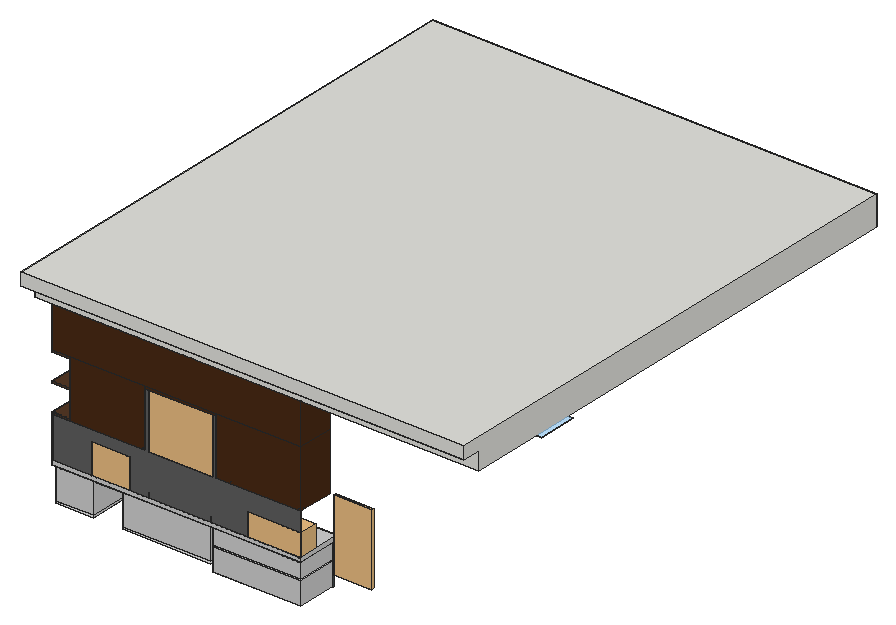
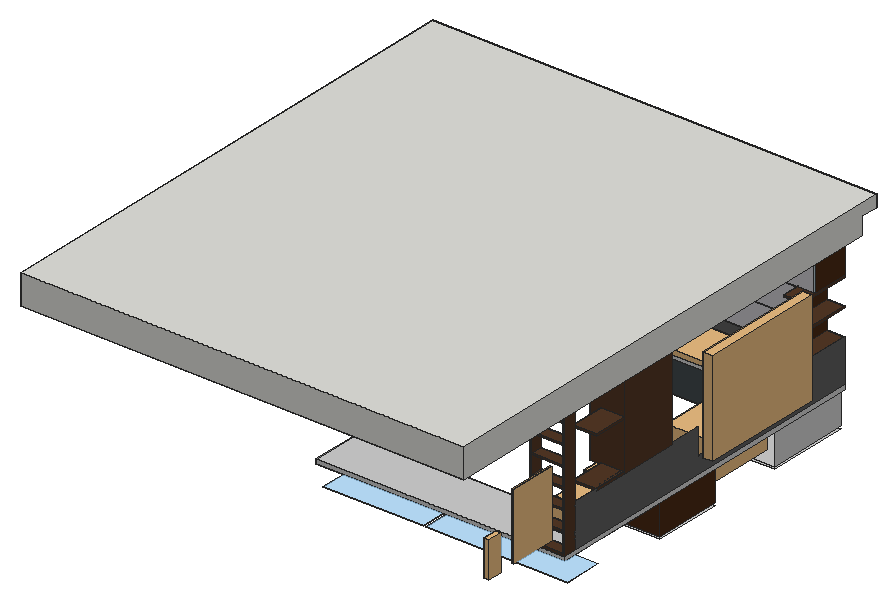
# SketchUp Ruby script. Lengths in inches.
U = 1.inch
M = Sketchup.active_model
def pt(a) = Geom::Point3d.new(a.map { |v| v * U })
def face(e, loops, mat)
  f = e.add_face(loops[0].map { |a| pt(a) })
  loops[1..].each { |l| e.add_face(l.map { |a| pt(a) }).erase! }
  f.material = f.back_material = mat if mat
  f
end
# faces: each face lists its corners as indices into pts; further lists are holes
def faces(e, pts, list, mat = nil) = list.each { |f| face(e, (f[0].is_a?(Array) ? f : [f]).map { |l| l.map { |i| pts[i] } }, mat) }
# xy, xz, yz: faces in a plane at the given z, y or x. An outline is a flat list of corners, or four numbers for a rectangle; further outlines are holes
def ring(l) = l.size == 4 ? [[l[0], l[1]], [l[2], l[1]], [l[2], l[3]], [l[0], l[3]]] : l.each_slice(2).to_a
def flat(e, list, mat, &to3) = list.each { |f| face(e, (f[0].is_a?(Array) ? f : [f]).map { |l| ring(l).map { |u, v| to3.(u, v) } }, mat) }
def xy(e, z, list, mat = nil) = flat(e, list, mat) { |x, y| [x, y, z] }
def xz(e, y, list, mat = nil) = flat(e, list, mat) { |x, z| [x, y, z] }
def yz(e, x, list, mat = nil) = flat(e, list, mat) { |y, z| [x, y, z] }
def lines(e, pts, list) = list.each { |a, b| e.add_line(pt(pts[a]), pt(pts[b])) }
# prism: a flat outline (further loops are holes) pulled along v
def prism(e, loops, v, mat = nil)
  f = face(e, loops, mat); d = Geom::Vector3d.new(v.map { |x| x * U })
  f.pushpull(f.normal.samedirection?(d) ? d.length : -d.length)
end
def box(e, o, s, mat = nil) = prism(e, [[o, [o[0] + s[0], o[1], o[2]], [o[0] + s[0], o[1] + s[1], o[2]], [o[0], o[1] + s[1], o[2]]]], [0, 0, s[2]], mat)
def at(x, y, z, deg = 0) = Geom::Transformation.translation(pt([x, y, z])) * Geom::Transformation.rotation(ORIGIN, Z_AXIS, deg.degrees)
def axes(o, x, y, z) = Geom::Transformation.new([*x, 0, *y, 0, *z, 0, *pt(o).to_a, 1])
def part(name) = M.definitions.add(name)
# library, detail: a bought-in or finely detailed component or shape, given as its bounding box
def library(name, o, s) = part(name).tap { |d| box(d.entities, o, s) }
def detail(e, o, s) = box(e.add_group.entities, o, s)
def put(e, d, t, mat = nil) = e.add_instance(d, t).tap { |i| i.material = mat if mat }
def group(e, t, mat = nil) = e.add_group.tap { |g| g.transformation = t; g.material = mat if mat }.entities
root = M.entities
M.materials.add("1472 AP 9469 Black Sea").color = [67, 75, 78]
M.materials.add("1474 AP 8274 WATER_S EDGE").color = [180, 198, 204]
M.materials.add("1513 AP K108 Rose Silver-N").color = [202, 201, 205]
M.materials.add("Counter Below Light").color = [252, 220, 183]
M.materials.add("Cupboard Light").color = [253, 210, 172]
M.materials.add("[Carrera Marble]").color = [207, 207, 207]
M.materials.add("[Stone Vein Gray]").color = [94, 94, 94]
M.materials.add("[Translucent Glass Blue]").color = [163, 215, 254]
M.materials["[Translucent Glass Blue]"].alpha = 0.5
M.materials.add("[Wood Veneer 01]").color = [83, 56, 38]
M.materials.add("[Wood Veneer 01]1").color = [74, 43, 22]
M.materials.add("[Wood Veneer 01]2").color = [120, 70, 37]
c1 = part("5")
box(c1.entities,[0,-0.25,-0.25],[0.5,45,11.6875])
c2 = part("6")
box(c2.entities,[0,-0.25,-0.25],[0.5,45,15.9375])
c3 = library("Group\#13",[0,0,0],[23.39,15.89,14.65])
c4 = library("Drawer fronts",[0,0,0],[1.57,26.54,41.66])
c5 = part("1")
box(c5.entities,[-20,0,0],[20,51,0.39])
c6 = library("Kitchen+Sink",[0,0,-9.45],[39.37,19.69,22.29])
c7 = library("ILVE HP75C",[-22.61,-16.47,-1.74],[45.22,32.94,3.48])
c8 = library("kitchen+utensil",[-39.88,-27.4,0],[79.77,28.4,32.96])
c9 = library("1\#1",[-14.37,-13.42,0],[27.79,27.79,26.46])
c10 = library("ACCESS \#17",[0,0,0],[12.33,19.09,15.22])
c11 = library("Kitchen Tray Decor",[57.57,5.21,10.61],[18.31,18.31,13.72])
c12 = library("Mi & Gei Hardware - Brass Towel Ring",[0,0,0],[7.7,2.76,18.21])
c13 = library("AS-120-mm",[0,0,0],[63,4.72,48])
c14 = library("Group\#79",[0,-1,0],[23.9375,1,23.9375])
c15 = part("8")
box(c15.entities,[0,-0.25,-0.25],[0.5,41.5,13.5])
c16 = part("Group\#68")
box(c16.entities,[0,0,0],[1,37.5,0.5])
c17 = library("angular chimney",[0,0,0],[18.55,32.4,33.35])
c18 = part("Group\#67")
box(c18.entities,[0,0,0],[28,1,0.5])
c19 = library("DC3A\#1",[-17.72,-4.29,0],[35.44,8.58,13.65])
c20 = library("oats",[14.82,-39.71,51.49],[19.78,4.73,8.06])
c21 = library("11",[-1.9375,-1.9375,-28],[4,4,28])
c22 = part("7")
xy(c22.entities,-1.25,[[0,-0.25,0.5,20.42],[0,20.52,0.5,41.08]])
xy(c22.entities,19.25,[[0,-0.25,0.5,20.42],[0,20.52,0.5,41.08]])
xz(c22.entities,-0.25,[[0,-1.25,0.5,19.25]])
xz(c22.entities,20.42,[[0,-1.25,0.5,19.25]])
xz(c22.entities,20.52,[[0,-1.25,0.5,19.25]])
xz(c22.entities,41.08,[[0,-1.25,0.5,19.25]])
yz(c22.entities,0,[[-0.25,-1.25,20.42,19.25],[20.52,-1.25,41.08,19.25]])
yz(c22.entities,0.5,[[-0.25,-1.25,20.42,19.25],[20.52,-1.25,41.08,19.25]],"1513 AP K108 Rose Silver-N")
p = [[0,20.52,0],[0,20.42,0],[0,20.42,19],[0,20.52,19]]
lines(c22.entities,p,[[0,1],[2,3]])
c23 = library("10",[-5.85,-5.85,-6.32],[15.7,15.7,6.32])
c24 = part("Group282\#1")
box(c24.entities,[-102,-4.5,0],[1,9,0.5])
c25 = part("Group283\#1")
box(c25.entities,[-100.5,-4.5,0],[1,9,0.5])
c26 = part("Group284\#1")
box(c26.entities,[-99,-4.5,0],[1,9,0.5])
c27 = part("Group285\#1")
box(c27.entities,[-97.5,-4.5,0],[1,9,0.5])
c28 = part("Group286\#1")
box(c28.entities,[-96,-4.5,0],[1,9,0.5])
c29 = part("Group287\#1")
box(c29.entities,[-94.5,-4.5,0],[1,9,0.5])
c30 = part("Group288\#1")
box(c30.entities,[-93,-4.5,0],[1,9,0.5])
c31 = part("Group289\#1")
box(c31.entities,[-91.5,-4.5,0],[1,9,0.5])
c32 = part("Group290\#1")
box(c32.entities,[-90,-4.5,0],[1,9,0.5])
c33 = part("Group291\#1")
box(c33.entities,[-88.5,-4.5,0],[1,9,0.5])
c34 = part("Group292\#1")
box(c34.entities,[-87,-4.5,0],[1,9,0.5])
c35 = part("Group293\#1")
box(c35.entities,[-85.5,-4.5,0],[1,9,0.5])
c36 = part("Group294\#1")
box(c36.entities,[-84,-4.5,0],[1,9,0.5])
c37 = part("Group295\#1")
box(c37.entities,[-82.5,-4.5,0],[1,9,0.5])
c38 = part("Group296\#1")
box(c38.entities,[-81,-4.5,0],[1,9,0.5])
c39 = part("Group297\#1")
box(c39.entities,[-79.5,-4.5,0],[1,9,0.5])
c40 = part("Group298\#1")
box(c40.entities,[-78,-4.5,0],[1,9,0.5])
c41 = part("Group299\#1")
box(c41.entities,[-76.5,-4.5,0],[1,9,0.5])
c42 = part("Group300\#1")
box(c42.entities,[-75,-4.5,0],[1,9,0.5])
c43 = part("Group301\#1")
box(c43.entities,[-73.5,-4.5,0],[1,9,0.5])
c44 = part("Group302\#1")
box(c44.entities,[-72,-4.5,0],[1,9,0.5])
c45 = part("Group303\#1")
box(c45.entities,[-70.5,-4.5,0],[1,9,0.5])
c46 = part("Group304\#1")
box(c46.entities,[-69,-4.5,0],[1,9,0.5])
c47 = part("Group305\#1")
box(c47.entities,[-67.5,-4.5,0],[1,9,0.5])
c48 = part("Group306\#1")
box(c48.entities,[-66,-4.5,0],[1,9,0.5])
c49 = part("Group307\#1")
box(c49.entities,[-64.5,-4.5,0],[1,9,0.5])
c50 = part("Group308\#1")
box(c50.entities,[-63,-4.5,0],[1,9,0.5])
c51 = part("Group309\#1")
box(c51.entities,[-61.5,-4.5,0],[1,9,0.5])
c52 = part("Group310\#1")
box(c52.entities,[-60,-4.5,0],[1,9,0.5])
c53 = part("Group311\#1")
box(c53.entities,[-58.5,-4.5,0],[1,9,0.5])
c54 = part("Group312\#1")
box(c54.entities,[-57,-4.5,0],[1,9,0.5])
c55 = part("Group313\#1")
box(c55.entities,[-55.5,-4.5,0],[1,9,0.5])
c56 = part("Group314\#1")
box(c56.entities,[-54,-4.5,0],[1,9,0.5])
c57 = part("Group315\#1")
box(c57.entities,[-52.5,-4.5,0],[1,9,0.5])
c58 = part("Group316\#1")
box(c58.entities,[-51,-4.5,0],[1,9,0.5])
c59 = part("Group317\#1")
box(c59.entities,[-49.5,-4.5,0],[1,9,0.5])
c60 = part("Group318\#1")
box(c60.entities,[-48,-4.5,0],[1,9,0.5])
c61 = part("Group319\#1")
box(c61.entities,[-46.5,-4.5,0],[1,9,0.5])
c62 = part("Group320\#1")
box(c62.entities,[-45,-4.5,0],[1,9,0.5])
c63 = part("Group321\#1")
box(c63.entities,[-43.5,-4.5,0],[1,9,0.5])
c64 = part("Group322\#1")
box(c64.entities,[-42,-4.5,0],[1,9,0.5])
c65 = part("Group323\#1")
box(c65.entities,[-40.5,-4.5,0],[1,9,0.5])
c66 = part("Group324\#1")
box(c66.entities,[-39,-4.5,0],[1,9,0.5])
c67 = part("Group325\#1")
box(c67.entities,[-37.5,-4.5,0],[1,9,0.5])
c68 = part("Group326\#1")
box(c68.entities,[-36,-4.5,0],[1,9,0.5])
c69 = part("Group327\#1")
box(c69.entities,[-34.5,-4.5,0],[1,9,0.5])
c70 = part("Group328\#1")
box(c70.entities,[-33,-4.5,0],[1,9,0.5])
c71 = part("Group329\#1")
box(c71.entities,[-31.5,-4.5,0],[1,9,0.5])
c72 = part("Group330\#1")
box(c72.entities,[-30,-4.5,0],[1,9,0.5])
c73 = part("Group331\#1")
box(c73.entities,[-28.5,-4.5,0],[1,9,0.5])
c74 = part("Group332\#1")
box(c74.entities,[-27,-4.5,0],[1,9,0.5])
c75 = part("Group333\#1")
box(c75.entities,[-25.5,-4.5,0],[1,9,0.5])
c76 = part("Group334\#1")
box(c76.entities,[-24,-4.5,0],[1,9,0.5])
c77 = part("Group335\#1")
box(c77.entities,[-22.5,-4.5,0],[1,9,0.5])
c78 = part("Group336\#1")
box(c78.entities,[-21,-4.5,0],[1,9,0.5])
c79 = part("Group337\#1")
box(c79.entities,[-19.5,-4.5,0],[1,9,0.5])
c80 = part("Group338\#1")
box(c80.entities,[-18,-4.5,0],[1,9,0.5])
c81 = part("Group339\#1")
box(c81.entities,[-16.5,-4.5,0],[1,9,0.5])
c82 = part("Group340\#1")
box(c82.entities,[-15,-4.5,0],[1,9,0.5])
c83 = part("Group341\#1")
box(c83.entities,[-13.5,-4.5,0],[1,9,0.5])
c84 = part("Group342\#1")
box(c84.entities,[-12,-4.5,0],[1,9,0.5])
c85 = part("Group343\#1")
box(c85.entities,[-10.5,-4.5,0],[1,9,0.5])
c86 = part("Group344\#1")
box(c86.entities,[-9,-4.5,0],[1,9,0.5])
c87 = part("Group345\#1")
box(c87.entities,[-7.5,-4.5,0],[1,9,0.5])
c88 = part("Group346\#1")
box(c88.entities,[-6,-4.5,0],[1,9,0.5])
c89 = part("Group347\#1")
box(c89.entities,[-4.5,-4.5,0],[1,9,0.5])
c90 = part("Group348\#1")
box(c90.entities,[-3,-4.5,0],[1,9,0.5])
c91 = part("Group349\#1")
box(c91.entities,[-1.5,-4.5,0],[1,9,0.5])
c92 = part("Group350\#1")
box(c92.entities,[0,-4.5,0],[1,9,0.5])
c93 = part("Group351\#1")
box(c93.entities,[1.5,-4.5,0],[1,9,0.5])
c94 = part("Group352\#1")
box(c94.entities,[3,-4.5,0],[1,9,0.5])
c95 = part("Group353\#1")
box(c95.entities,[4.5,-4.5,0],[1,9,0.5])
c96 = part("Group354\#1")
box(c96.entities,[6,-4.5,0],[1,9,0.5])
c97 = part("Group355\#1")
box(c97.entities,[7.5,-4.5,0],[1,9,0.5])
c98 = part("Group356\#1")
box(c98.entities,[9,-4.5,0],[1,9,0.5])
c99 = part("Group357\#1")
box(c99.entities,[10.5,-4.5,0],[1,9,0.5])
c100 = part("Group358\#1")
box(c100.entities,[12,-4.5,0],[1,9,0.5])
c101 = part("Group359\#1")
box(c101.entities,[13.5,-4.5,0],[1,9,0.5])
c102 = part("Group360\#1")
box(c102.entities,[15,-4.5,0],[1,9,0.5])
c103 = part("Group361\#1")
box(c103.entities,[16.5,-4.5,0],[1,9,0.5])
c104 = part("Group362\#1")
box(c104.entities,[18,-4.5,0],[1,9,0.5])
c105 = part("Group363\#1")
box(c105.entities,[19.5,-4.5,0],[1,9,0.5])
c106 = part("Group364\#1")
box(c106.entities,[21,-4.5,0],[1,9,0.5])
c107 = part("Group365\#1")
box(c107.entities,[22.5,-4.5,0],[1,9,0.5])
c108 = part("Group366\#1")
box(c108.entities,[24,-4.5,0],[1,9,0.5])
c109 = part("Group367\#1")
box(c109.entities,[25.5,-4.5,0],[1,9,0.5])
c110 = part("Group368\#1")
box(c110.entities,[27,-4.5,0],[1,9,0.5])
c111 = part("Group369\#1")
box(c111.entities,[28.5,-4.5,0],[1,9,0.5])
c112 = part("Group370\#1")
box(c112.entities,[30,-4.5,0],[1,9,0.5])
c113 = part("Group371\#1")
box(c113.entities,[31.5,-4.5,0],[1,9,0.5])
c114 = part("Group372\#1")
box(c114.entities,[33,-4.5,0],[1,9,0.5])
c115 = part("Group373\#1")
box(c115.entities,[34.5,-4.5,0],[1,9,0.5])
c116 = part("Group374\#1")
box(c116.entities,[36,-4.5,0],[1,9,0.5])
c117 = part("Group375\#1")
box(c117.entities,[37.5,-4.5,0],[1,9,0.5])
c118 = part("Group376\#1")
box(c118.entities,[39,-4.5,0],[1,9,0.5])
c119 = part("Group377\#1")
box(c119.entities,[40.5,-4.5,0],[1,9,0.5])
c120 = part("Group378\#1")
box(c120.entities,[42,-4.5,0],[1,9,0.5])
c121 = part("Group379\#1")
box(c121.entities,[43.5,-4.5,0],[1,9,0.5])
c122 = part("Group380\#1")
box(c122.entities,[45,-4.5,0],[1,9,0.5])
c123 = part("Group381\#1")
box(c123.entities,[46.5,-4.5,0],[1,9,0.5])
c124 = part("Group382\#1")
box(c124.entities,[48,-4.5,0],[1,9,0.5])
c125 = part("Group383\#1")
box(c125.entities,[49.5,-4.5,0],[1,9,0.5])
c126 = part("Group384\#1")
box(c126.entities,[51,-4.5,0],[1,9,0.5])
c127 = part("Group385\#1")
box(c127.entities,[52.5,-4.5,0],[1,9,0.5])
c128 = part("Group386\#1")
box(c128.entities,[54,-4.5,0],[1,9,0.5])
c129 = part("Group387\#1")
box(c129.entities,[55.5,-4.5,0],[1,9,0.5])
c130 = part("Group388\#1")
box(c130.entities,[57,-4.5,0],[1,9,0.5])
c131 = part("Group389\#1")
box(c131.entities,[58.5,-4.5,0],[1,9,0.5])
c132 = part("Group390\#1")
box(c132.entities,[60,-4.5,0],[1,9,0.5])
c133 = part("Group391\#1")
box(c133.entities,[61.5,-4.5,0],[1,9,0.5])
c134 = part("Group392\#1")
box(c134.entities,[63,-4.5,0],[1,9,0.5])
c135 = part("Group393\#1")
box(c135.entities,[64.5,-4.5,0],[1,9,0.5])
c136 = part("Group394\#1")
box(c136.entities,[66,-4.5,0],[1,9,0.5])
c137 = part("Group395\#1")
box(c137.entities,[67.5,-4.5,0],[1,9,0.5])
c138 = part("Group396\#1")
box(c138.entities,[69,-4.5,0],[1,9,0.5])
c139 = part("Group397\#1")
box(c139.entities,[70.5,-4.5,0],[1,9,0.5])
c140 = part("Group398\#1")
box(c140.entities,[72,-4.5,0],[1,9,0.5])
c141 = part("Group399\#1")
box(c141.entities,[73.5,-4.5,0],[1,9,0.5])
c142 = part("Group400\#1")
box(c142.entities,[75,-4.5,0],[1,9,0.5])
c143 = part("Group401\#1")
box(c143.entities,[76.5,-4.5,0],[1,9,0.5])
c144 = part("Group402\#1")
box(c144.entities,[78,-4.5,0],[1,9,0.5])
c145 = part("Group403\#1")
box(c145.entities,[79.5,-4.5,0],[1,9,0.5])
c146 = part("Group404\#1")
box(c146.entities,[81,-4.5,0],[1,9,0.5])
c147 = part("Group405\#1")
box(c147.entities,[82.5,-4.5,0],[1,9,0.5])
c148 = part("Group406\#1")
box(c148.entities,[84,-4.5,0],[1,9,0.5])
c149 = part("Group407\#1")
box(c149.entities,[85.5,-4.5,0],[1,9,0.5])
c150 = part("Group408\#1")
box(c150.entities,[87,-4.5,0],[1,9,0.5])
c151 = part("Group409\#1")
box(c151.entities,[88.5,-4.5,0],[1,9,0.5])
c152 = part("Group410\#1")
box(c152.entities,[90,-4.5,0],[1,9,0.5])
c153 = part("Group411\#1")
box(c153.entities,[91.5,-4.5,0],[1,9,0.5])
c154 = part("Group412\#1")
box(c154.entities,[93,-4.5,0],[1,9,0.5])
c155 = part("Group413\#1")
box(c155.entities,[94.5,-4.5,0],[1,9,0.5])
c156 = part("Group414\#1")
box(c156.entities,[96,-4.5,0],[1,9,0.5])
c157 = part("Group415\#1")
box(c157.entities,[97.5,-4.5,0],[1,9,0.5])
c158 = part("Group416\#1")
box(c158.entities,[99,-4.5,0],[1,9,0.5])
c159 = part("Group417\#1")
box(c159.entities,[100.5,-4.5,0],[1,9,0.5])
c160 = part("Group280\#1")
put(c160.entities,c24,at(0,0,0))
put(c160.entities,c25,at(0,0,0))
put(c160.entities,c26,at(0,0,0))
put(c160.entities,c27,at(0,0,0))
put(c160.entities,c28,at(0,0,0))
put(c160.entities,c29,at(0,0,0))
put(c160.entities,c30,at(0,0,0))
put(c160.entities,c31,at(0,0,0))
put(c160.entities,c32,at(0,0,0))
put(c160.entities,c33,at(0,0,0))
put(c160.entities,c34,at(0,0,0))
put(c160.entities,c35,at(0,0,0))
put(c160.entities,c36,at(0,0,0))
put(c160.entities,c37,at(0,0,0))
put(c160.entities,c38,at(0,0,0))
put(c160.entities,c39,at(0,0,0))
put(c160.entities,c40,at(0,0,0))
put(c160.entities,c41,at(0,0,0))
put(c160.entities,c42,at(0,0,0))
put(c160.entities,c43,at(0,0,0))
put(c160.entities,c44,at(0,0,0))
put(c160.entities,c45,at(0,0,0))
put(c160.entities,c46,at(0,0,0))
put(c160.entities,c47,at(0,0,0))
put(c160.entities,c48,at(0,0,0))
put(c160.entities,c49,at(0,0,0))
put(c160.entities,c50,at(0,0,0))
put(c160.entities,c51,at(0,0,0))
put(c160.entities,c52,at(0,0,0))
put(c160.entities,c53,at(0,0,0))
put(c160.entities,c54,at(0,0,0))
put(c160.entities,c55,at(0,0,0))
put(c160.entities,c56,at(0,0,0))
put(c160.entities,c57,at(0,0,0))
put(c160.entities,c58,at(0,0,0))
put(c160.entities,c59,at(0,0,0))
put(c160.entities,c60,at(0,0,0))
put(c160.entities,c61,at(0,0,0))
put(c160.entities,c62,at(0,0,0))
put(c160.entities,c63,at(0,0,0))
put(c160.entities,c64,at(0,0,0))
put(c160.entities,c65,at(0,0,0))
put(c160.entities,c66,at(0,0,0))
put(c160.entities,c67,at(0,0,0))
put(c160.entities,c68,at(0,0,0))
put(c160.entities,c69,at(0,0,0))
put(c160.entities,c70,at(0,0,0))
put(c160.entities,c71,at(0,0,0))
put(c160.entities,c72,at(0,0,0))
put(c160.entities,c73,at(0,0,0))
put(c160.entities,c74,at(0,0,0))
put(c160.entities,c75,at(0,0,0))
put(c160.entities,c76,at(0,0,0))
put(c160.entities,c77,at(0,0,0))
put(c160.entities,c78,at(0,0,0))
put(c160.entities,c79,at(0,0,0))
put(c160.entities,c80,at(0,0,0))
put(c160.entities,c81,at(0,0,0))
put(c160.entities,c82,at(0,0,0))
put(c160.entities,c83,at(0,0,0))
put(c160.entities,c84,at(0,0,0))
put(c160.entities,c85,at(0,0,0))
put(c160.entities,c86,at(0,0,0))
put(c160.entities,c87,at(0,0,0))
put(c160.entities,c88,at(0,0,0))
put(c160.entities,c89,at(0,0,0))
put(c160.entities,c90,at(0,0,0))
put(c160.entities,c91,at(0,0,0))
put(c160.entities,c92,at(0,0,0))
put(c160.entities,c93,at(0,0,0))
put(c160.entities,c94,at(0,0,0))
put(c160.entities,c95,at(0,0,0))
put(c160.entities,c96,at(0,0,0))
put(c160.entities,c97,at(0,0,0))
put(c160.entities,c98,at(0,0,0))
put(c160.entities,c99,at(0,0,0))
put(c160.entities,c100,at(0,0,0))
put(c160.entities,c101,at(0,0,0))
put(c160.entities,c102,at(0,0,0))
put(c160.entities,c103,at(0,0,0))
put(c160.entities,c104,at(0,0,0))
put(c160.entities,c105,at(0,0,0))
put(c160.entities,c106,at(0,0,0))
put(c160.entities,c107,at(0,0,0))
put(c160.entities,c108,at(0,0,0))
put(c160.entities,c109,at(0,0,0))
put(c160.entities,c110,at(0,0,0))
put(c160.entities,c111,at(0,0,0))
put(c160.entities,c112,at(0,0,0))
put(c160.entities,c113,at(0,0,0))
put(c160.entities,c114,at(0,0,0))
put(c160.entities,c115,at(0,0,0))
put(c160.entities,c116,at(0,0,0))
put(c160.entities,c117,at(0,0,0))
put(c160.entities,c118,at(0,0,0))
put(c160.entities,c119,at(0,0,0))
put(c160.entities,c120,at(0,0,0))
put(c160.entities,c121,at(0,0,0))
put(c160.entities,c122,at(0,0,0))
put(c160.entities,c123,at(0,0,0))
put(c160.entities,c124,at(0,0,0))
put(c160.entities,c125,at(0,0,0))
put(c160.entities,c126,at(0,0,0))
put(c160.entities,c127,at(0,0,0))
put(c160.entities,c128,at(0,0,0))
put(c160.entities,c129,at(0,0,0))
put(c160.entities,c130,at(0,0,0))
put(c160.entities,c131,at(0,0,0))
put(c160.entities,c132,at(0,0,0))
put(c160.entities,c133,at(0,0,0))
put(c160.entities,c134,at(0,0,0))
put(c160.entities,c135,at(0,0,0))
put(c160.entities,c136,at(0,0,0))
put(c160.entities,c137,at(0,0,0))
put(c160.entities,c138,at(0,0,0))
put(c160.entities,c139,at(0,0,0))
put(c160.entities,c140,at(0,0,0))
put(c160.entities,c141,at(0,0,0))
put(c160.entities,c142,at(0,0,0))
put(c160.entities,c143,at(0,0,0))
put(c160.entities,c144,at(0,0,0))
put(c160.entities,c145,at(0,0,0))
put(c160.entities,c146,at(0,0,0))
put(c160.entities,c147,at(0,0,0))
put(c160.entities,c148,at(0,0,0))
put(c160.entities,c149,at(0,0,0))
put(c160.entities,c150,at(0,0,0))
put(c160.entities,c151,at(0,0,0))
put(c160.entities,c152,at(0,0,0))
put(c160.entities,c153,at(0,0,0))
put(c160.entities,c154,at(0,0,0))
put(c160.entities,c155,at(0,0,0))
put(c160.entities,c156,at(0,0,0))
put(c160.entities,c157,at(0,0,0))
put(c160.entities,c158,at(0,0,0))
put(c160.entities,c159,at(0,0,0))
xy(root,17.25,[[89.5,10,134,30]],"[Carrera Marble]")
xy(root,20.5,[[10,10,29,52],[44,10,88.5,30],[10,89.5,30,124.5]],"[Carrera Marble]")
xy(root,21.5,[[10,10,29,52],[44,10,88.5,30]],"[Carrera Marble]")
xy(root,21.5,[[10,89.5,30,124.5]],"[Wood Veneer 01]1")
xy(root,28.4375,[[89.5,10,134,30]],"[Carrera Marble]")
xy(root,29.4375,[[89.5,10,134,30]],"[Carrera Marble]")
xy(root,36.9375,[[10,10,10,52,30,52,30,31,29,31,29,10],[31,10,43,30],[44,10,88.5,30],[89.5,10,134,30],[[10,53,30,88.5],[12,56,28,85.5]],
  [10,89.5,30,124.5],[10,125.5,30,161],[31,162,31,163,10,163,10,183,82,183,82,162],[83,162,134,183]],"[Carrera Marble]")
xy(root,38,[[[9,9,135,9,135,30,30,30,30,162,135,162,135,186,134,186,134,184.5,10,184.5,10,186,9,186],[12,56,28,85.5]]],"[Carrera Marble]")
xy(root,111,[[[0,9,225,261],[9,30,213,252]]])
xy(root,120,[[0,0,225,9],[[9,30,213,252],[45,66,45.004,66,45,66.063]],[45,66,45,66.063,45.004,66]])
xy(root,126,[[0,0,225,261]])
xz(root,0,[[0,120,225,126]])
xz(root,9,[[0,111,225,120]])
xz(root,10,[[89.5,17.25,134,28.4375],[10,21.5,29,36.9375],[44,21.5,88.5,36.9375],[89.5,29.4375,134,36.9375]],"[Carrera Marble]")
xz(root,30,[[9,111,213,120]])
xz(root,56,[[12,36.9375,28,38]],"[Carrera Marble]")
xz(root,85.5,[[12,36.9375,28,38]],"[Carrera Marble]")
xz(root,89.5,[[10,21.5,30,36.9375]],"[Wood Veneer 01]1")
xz(root,124.5,[[10,21.5,30,36.9375]],"[Wood Veneer 01]1")
xz(root,252,[[9,111,213,120]])
xz(root,261,[[0,111,225,126]])
yz(root,0,[[9,111,9,120,0,120,0,126,261,126,261,111]])
yz(root,9,[[30,111,252,120]])
yz(root,10,[[10,21.5,52,36.9375]],"[Carrera Marble]")
yz(root,10,[[89.5,21.5,124.5,36.9375]],"[Wood Veneer 01]1")
yz(root,12,[[56,36.9375,85.5,38]],"[Carrera Marble]")
yz(root,28,[[56,36.9375,85.5,38]],"[Carrera Marble]")
yz(root,29,[[10,20.5,31,21.5],[31,20.5,52,21.5],[10,21.5,31,36.9375]],"[Carrera Marble]")
yz(root,44,[[10,21.5,30,36.9375]],"[Carrera Marble]")
yz(root,88.5,[[10,21.5,30,36.9375]],"[Carrera Marble]")
yz(root,89.5,[[10,17.25,30,28.4375],[10,29.4375,30,36.9375]],"[Carrera Marble]")
yz(root,134,[[10,17.25,30,28.4375],[10,29.4375,30,36.9375]],"[Carrera Marble]")
yz(root,213,[[30,111,252,120]])
yz(root,225,[[9,111,261,111,261,126,0,126,0,120,9,120]])
put(root,c1,at(134,30,17.25,90),"1472 AP 9469 Black Sea")
put(root,c2,at(88.5,30,21.5,90),"1472 AP 9469 Black Sea")
put(root,c3,axes([30,91.625,21.5],[0,1.33,0],[-1,0,0],[0,0,1.05407]),"[Carrera Marble]")
put(root,c4,axes([155,28.71,23.79],[0,0.82,0],[-0.71577,0,0],[0,0,0.8692]),"[Carrera Marble]")
put(root,c5,axes([134,183,26.03],[0,1,0],[-1,0,0],[0,0,1.0625]),"[Translucent Glass Blue]")
put(root,c5,axes([82,183,26.03],[0,1,0],[-1.41176,0,0],[0,0,1.0625]),"[Translucent Glass Blue]")
g1 = group(root,at(134,30,29.4375,90),"1472 AP 9469 Black Sea")
box(g1,[0,-0.25,-0.25],[0.5,45,8])
put(root,c6,at(30.47,55.68,40,90),"[Carrera Marble]")
g2 = group(root,at(135,9,38,90),"[Carrera Marble]")
xy(g2,0,[[[0,0,0,126,177,126,177,0,151,0,151,103,23,103,23,0],[47,104.53,76.5,124.16],[176,1.25,176.5,124.75]]])
xy(g2,0.5,[[176,1.25,176.5,124.75]])
xy(g2,1.5,[[76.5,104.53,85.875,124.16]])
xy(g2,2,[[[0,0,23,0,23,103,151,103,151,0,177,0,177,126,0,126],[47,104.53,85.875,124.16]]])
xz(g2,0,[[0,0,23,2],[151,0,177,2]])
xz(g2,1.25,[[176,0,176.5,0.5]])
xz(g2,103,[[23,0,151,2]])
xz(g2,104.53,[[47,0,47,2,85.875,2,85.875,1.5,76.5,1.5,76.5,0]])
xz(g2,124.16,[[47,0,76.5,0,76.5,1.5,85.875,1.5,85.875,2,47,2]])
xz(g2,124.75,[[176,0,176.5,0.5]])
xz(g2,126,[[0,0,177,2]])
yz(g2,0,[[0,0,126,2]])
yz(g2,23,[[0,0,103,2]])
yz(g2,47,[[104.53,0,124.16,2]])
yz(g2,76.5,[[104.53,0,124.16,1.5]])
yz(g2,85.875,[[104.53,1.5,124.16,2]])
yz(g2,151,[[0,0,103,2]])
yz(g2,176,[[1.25,0,124.75,0.5]])
yz(g2,176.5,[[1.25,0,124.75,0.5]])
yz(g2,177,[[0,0,126,2]])
g3 = group(g2,at(176,1.25,0),"Counter Below Light")
box(g3,[0,0,0],[0.5,123.5,0.5])
g4 = group(root,at(9,185,40,90),"[Wood Veneer 01]")
xy(g4,0,[[-5,-18,1,0]])
xy(g4,1,[[-5,-17,1,-1]])
xy(g4,10.86,[[-5,-17,1,-1]])
xy(g4,11.36,[[-5,-17,1,-1]])
xy(g4,20.71,[[-5,-17,1,-1]])
xy(g4,21.21,[[-5,-17,1,-1]])
xy(g4,30.57,[[-5,-17,1,-1]])
xy(g4,31.07,[[-5,-17,1,-1]])
xy(g4,40.43,[[-5,-17,1,-1]])
xy(g4,40.93,[[-5,-17,1,-1]])
xy(g4,50.29,[[-5,-17,1,-1]])
xy(g4,50.79,[[-5,-17,1,-1]])
xy(g4,60.14,[[-5,-17,1,-1]])
xy(g4,60.64,[[-5,-17,1,-1]])
xy(g4,70,[[-5,-17,1,-1]])
xy(g4,71,[[-5,-18,1,0]])
xz(g4,-18,[[-5,0,1,71]])
xz(g4,-17,[[-5,1,1,10.86],[-5,11.36,1,20.71],[-5,21.21,1,30.57],[-5,31.07,1,40.43],[-5,40.93,1,50.29],
  [-5,50.79,1,60.14],[-5,60.64,1,70]])
xz(g4,-1,[[-5,1,1,10.86],[-5,11.36,1,20.71],[-5,21.21,1,30.57],[-5,31.07,1,40.43],[-5,40.93,1,50.29],
  [-5,50.79,1,60.14],[-5,60.64,1,70]])
xz(g4,0,[[-5,0,1,71]])
yz(g4,-5,[[[-18,0,0,71],[-17,21.21,-1,21.21,-1,30.57,-17,30.57,-17,31.07,-1,31.07,-1,40.43,-17,40.43,-17,40.93,-1,40.93,-1,50.29,-17,50.29,-17,50.79,-1,50.79,-1,60.14,-17,60.14],[-17,1,-1,10.86],[-17,60.64,-1,70],[-17,11.36,-1,20.71]]])
yz(g4,1,[[[-18,0,0,71],[-17,1,-1,10.86],[-17,60.64,-1,70],[-17,50.79,-1,60.14],[-17,40.93,-1,50.29],[-17,31.07,-1,40.43],[-17,11.36,-1,20.71],[-17,21.21,-1,30.57]]])
put(root,c7,axes([73.58,20.61,41.22],[0.7,0,0],[0,-0.7,0],[0,0,0.7]))
put(root,c8,axes([121.44,9.42,40],[-0.34,0,0],[0,-0.34,0],[0,0,0.34]))
put(root,c9,axes([18.56,142.34,40],[0,0.66,0],[-0.66,0,0],[0,0,0.66]))
put(root,c10,axes([29.04,9.08,40],[0,1,0],[1,0,0],[0,0,1]))
put(root,c11,at(32.6,95.99,29.39,90))
g5 = group(root,at(135,9,40,90))
xy(g5,0,[[0,0,0.08,125.92],[0,125.92,171,126]],"[Stone Vein Gray]")
xy(g5,9,[[30,125.92,93,126]],"[Stone Vein Gray]")
xy(g5,22,[[0,0,0.08,43],[0,79,0.08,125.92],[0,125.92,30,126],[93,125.92,171,126]],"[Stone Vein Gray]")
xy(g5,49,[[0,43,0.08,79]],"[Stone Vein Gray]")
xz(g5,0,[[0,0,0.08,22]],"[Stone Vein Gray]")
xz(g5,43,[[0,22,0.08,49]],"[Stone Vein Gray]")
xz(g5,79,[[0,22,0.08,49]],"[Stone Vein Gray]")
xz(g5,125.92,[[0.08,0,171,0,171,22,93,22,93,9,30,9,30,22,0.08,22]],"[Stone Vein Gray]")
xz(g5,126,[[0,0,0,22,30,22,30,9,93,9,93,22,171,22,171,0]],"[Stone Vein Gray]")
yz(g5,0.08,[[0,0,125.92,0,125.92,22,79,22,79,49,43,49,43,22,0,22]],"[Stone Vein Gray]")
yz(g5,30,[[125.92,9,126,22]],"[Stone Vein Gray]")
yz(g5,93,[[125.92,9,126,22]],"[Stone Vein Gray]")
yz(g5,171,[[125.92,0,126,22]],"[Stone Vein Gray]")
put(root,c12,at(15.4,221.93,47.19,90))
put(root,c13,axes([1.4,39,49],[0,1,0],[1,0,0],[0,0,1]))
put(root,c14,axes([10,193.03,49.95],[0,1,0],[-1,0,0],[0,0,1.4]))
g6 = group(root,at(135,9,61,90),"[Wood Veneer 01]1")
xy(g6,0,[[0,0,0,43,18,43,18,0,2,0,2,42.5,1,42.5,1,0],[0,79,0,117,1,117,1,79.5,2,79.5,2,117,18,117,18,79]])
xy(g6,0.5,[[1,0,2,42.5],[1,79.5,2,117]])
xy(g6,1,[[1,80,18,97.5],[1,98.5,18,116]])
xy(g6,1,[[1,1,18,21],[1,22,18,42]],"[Wood Veneer 01]")
xy(g6,14,[[1,1,18,21],[1,22,18,42],[1,80,18,97.5],[1,98.5,18,116]])
xy(g6,15,[[1,1,18,42],[1,80,18,116]])
xy(g6,28,[[1,1,18,42],[0,43,18,79],[1,80,18,116]])
xy(g6,29,[[0,0,18,117]])
xz(g6,0,[[0,0,1,0,1,0.5,2,0.5,2,0,18,0,18,29,0,29]])
xz(g6,1,[[1,15,18,28]])
xz(g6,1,[[1,1,18,14]],"[Wood Veneer 01]")
xz(g6,21,[[1,1,18,14]],"[Wood Veneer 01]")
xz(g6,22,[[1,1,18,14]],"[Wood Veneer 01]")
xz(g6,42,[[1,15,18,28]])
xz(g6,42,[[1,1,18,14]],"[Wood Veneer 01]")
xz(g6,42.5,[[1,0,2,0.5]])
xz(g6,43,[[0,0,18,28]])
xz(g6,79,[[0,0,18,28]])
xz(g6,79.5,[[1,0,2,0.5]])
xz(g6,80,[[1,1,18,14],[1,15,18,28]])
xz(g6,97.5,[[1,1,18,14]])
xz(g6,98.5,[[1,1,18,14]])
xz(g6,116,[[1,1,18,14],[1,15,18,28]])
xz(g6,117,[[0,0,0,29,18,29,18,0,2,0,2,0.5,1,0.5,1,0]])
yz(g6,0,[[0,0,43,29],[79,0,79,28,43,28,43,29,117,29,117,0]])
yz(g6,1,[[0,0,42.5,0.5],[79.5,0,117,0.5],[80,1,97.5,14],[98.5,1,116,14],[1,15,42,28],
  [80,15,116,28]])
yz(g6,1,[[1,1,21,14],[22,1,42,14]],"[Wood Veneer 01]")
yz(g6,2,[[0,0,42.5,0.5],[79.5,0,117,0.5]])
yz(g6,18,[[[0,0,43,0,43,28,79,28,79,0,117,0,117,29,0,29],[1,15,42,28],[80,15,116,28],[80,1,80,14,97.5,14,97.5,1,98.5,1,98.5,14,116,14,116,1],[1,1,21,14],[22,1,42,14]]])
put(g6,c15,at(18,1,15),"1513 AP K108 Rose Silver-N")
put(g6,c15,axes([18,80,15],[1,0,0],[0,0.87805,0],[0,0,1]),"1513 AP K108 Rose Silver-N")
put(g6,c15,axes([18,80,1],[1,0,0],[0,0.87805,0],[0,0,1]),"1513 AP K108 Rose Silver-N")
g7 = group(g6,at(0,117,0),"[Wood Veneer 01]")
box(g7,[0,0,28],[27,9,1])
box(g7,[0,0,14],[27,9,1])
box(g7,[0,0,0],[27,9,1])
put(g6,c16,at(1,79.5,0),"Cupboard Light")
put(g6,c16,axes([1,0,0],[1,0,0],[0,1.13333,0],[0,0,1]),"Cupboard Light")
put(root,c17,axes([90.21,9.08,61],[0,0.99328,0],[-1,0,0],[0,0,0.83947]),"[Carrera Marble]")
g8 = group(root,at(9,118,61,90),"[Wood Veneer 01]")
xy(g8,0,[[0,-18,0,0,30,0,30,-1,0.5,-1,0.5,-2,30,-2,30,-18]])
xy(g8,0.5,[[0.5,-2,30,-1]])
xy(g8,1,[[1,-18,29,-1]])
xy(g8,16.5,[[1,-18,29,-7],[1,-6,29,-1]])
xy(g8,17,[[1,-7,29,-6]])
xy(g8,17.5,[[1,-18,29,-1]])
xy(g8,32.5,[[1,-18,29,-7],[1,-6,29,-1]])
xy(g8,33,[[1,-7,29,-6]])
xy(g8,33.5,[[1,-18,29,-1]])
xy(g8,49,[[1,-18,29,-7],[1,-6,29,-1]])
xy(g8,49.5,[[1,-7,29,-6]])
xy(g8,50,[[0,-18,30,0]])
xz(g8,-18,[[[0,0,30,50],[1,33.5,29,49],[1,1,29,16.5],[1,17.5,29,32.5]]])
xz(g8,-7,[[1,16.5,29,17],[1,32.5,29,33],[1,49,29,49.5]])
xz(g8,-6,[[1,16.5,29,17],[1,32.5,29,33],[1,49,29,49.5]])
xz(g8,-2,[[0.5,0,30,0.5]])
xz(g8,-1,[[0.5,0,30,0.5],[1,1,29,16.5],[1,17.5,29,32.5],[1,33.5,29,49]])
xz(g8,0,[[0,0,30,50]])
yz(g8,0,[[-18,0,0,50]])
yz(g8,0.5,[[-2,0,-1,0.5]])
yz(g8,1,[[-18,1,-1,1,-1,16.5,-6,16.5,-6,17,-7,17,-7,16.5,-18,16.5],[-18,17.5,-1,17.5,-1,32.5,-6,32.5,-6,33,-7,33,-7,32.5,-18,32.5],[-18,33.5,-1,33.5,-1,49,-6,49,-6,49.5,-7,49.5,-7,49,-18,49]])
yz(g8,29,[[-18,1,-18,16.5,-7,16.5,-7,17,-6,17,-6,16.5,-1,16.5,-1,1],[-18,17.5,-18,32.5,-7,32.5,-7,33,-6,33,-6,32.5,-1,32.5,-1,17.5],[-18,33.5,-18,49,-7,49,-7,49.5,-6,49.5,-6,49,-1,49,-1,33.5]])
yz(g8,30,[[-18,0,-2,0,-2,0.5,-1,0.5,-1,0,0,0,0,50,-18,50]])
g9 = group(g8,at(30,0,49.2))
box(g9,[0,-12,0],[18,12,0.8])
g10 = group(g8,at(36,0,25))
box(g10,[-6,-12,0],[18,12,0.8])
g11 = group(g8,at(30,0,0))
xy(g11,0,[[0,-12,0,-2,17.5,-2,17.5,-1,0,-1,0,0,18,0,18,-12]])
xy(g11,0.5,[[0,-2,17.5,-1]])
xy(g11,0.8,[[0,-12,18,0]])
xz(g11,-12,[[0,0,18,0.8]])
xz(g11,-2,[[0,0,17.5,0.5]])
xz(g11,-1,[[0,0,17.5,0.5]])
xz(g11,0,[[0,0,18,0.8]])
yz(g11,0,[[-12,0,-12,0.8,0,0.8,0,0,-1,0,-1,0.5,-2,0.5,-2,0]])
yz(g11,17.5,[[-2,0,-1,0.5]])
yz(g11,18,[[-12,0,0,0.8]])
put(g8,c18,at(1,-7,49),"Cupboard Light")
put(g8,c18,at(1,-7,32.5),"Cupboard Light")
put(g8,c18,at(1,-7,16.5),"Cupboard Light")
put(g8,c18,axes([0.5,-2,0],[1.67857,0,0],[0,1,0],[0,0,1]),"Cupboard Light")
put(root,c19,axes([102.94,22.48,62],[0.5612,0,0],[0,0.5612,0],[0,0,0.5612]))
put(root,c20,at(99.18,58.48,10.51),"[Carrera Marble]")
put(root,c21,at(126.65,178.01,112.83,90))
put(root,c21,at(108.65,178.01,112.83,90))
put(root,c21,at(90.65,178.01,112.83,90))
g12 = group(root,at(135,9,90,90),"[Wood Veneer 01]1")
xy(g12,0,[[0,0,0,126,18,126,18,125,1,125,1,84.17,18,84.17,18,83.17,1,83.17,1,42.83,18,42.83,18,41.83,1,41.83,1,1,18,1,18,0]])
xy(g12,20,[[1,1,18,41.83],[1,42.83,18,83.17],[1,84.17,18,125]])
xy(g12,21,[[0,0,18,126]])
xz(g12,0,[[0,0,18,21]])
xz(g12,1,[[1,0,18,20]])
xz(g12,41.83,[[1,0,18,20]])
xz(g12,42.83,[[1,0,18,20]])
xz(g12,83.17,[[1,0,18,20]])
xz(g12,84.17,[[1,0,18,20]])
xz(g12,125,[[1,0,18,20]])
xz(g12,126,[[0,0,18,21]])
yz(g12,0,[[0,0,126,21]])
yz(g12,1,[[1,0,41.83,20],[42.83,0,83.17,20],[84.17,0,125,20]])
yz(g12,18,[[0,0,1,0,1,20,41.83,20,41.83,0,42.83,0,42.83,20,83.17,20,83.17,0,84.17,0,84.17,20,125,20,125,0,126,0,126,21,0,21]])
put(g12,c22,at(18,1,1),"1474 AP 8274 WATER_S EDGE")
put(g12,c22,at(18,84.17,1),"1474 AP 8274 WATER_S EDGE")
put(g12,c22,axes([18,42.83,1],[1,0,0],[0,0.98776,0],[0,0,1]),"1474 AP 8274 WATER_S EDGE")
put(root,c23,at(185,56,112.61,90))
put(root,c23,at(41,56,112.61,90))
put(root,c23,at(89,52.01,112.61,90))
put(root,c23,at(137,52.01,112.61,90))
put(root,c23,axes([89,230.06,112.61],[0,-1,0],[-1,0,0],[0,0,1]))
put(root,c23,axes([137,230.06,112.61],[0,-1,0],[-1,0,0],[0,0,1]))
put(root,c23,at(35,111.35,112.61,90))
put(root,c23,at(191,111.35,112.61,90))
put(root,c23,at(35,166.71,112.61,90))
put(root,c23,at(191,166.71,112.61,90))
put(root,c23,at(185,222.0625,112.61,90))
put(root,c160,axes([111,30,115.5],[-1,0,0],[0,0,1],[0,1,0]),"[Wood Veneer 01]2")
